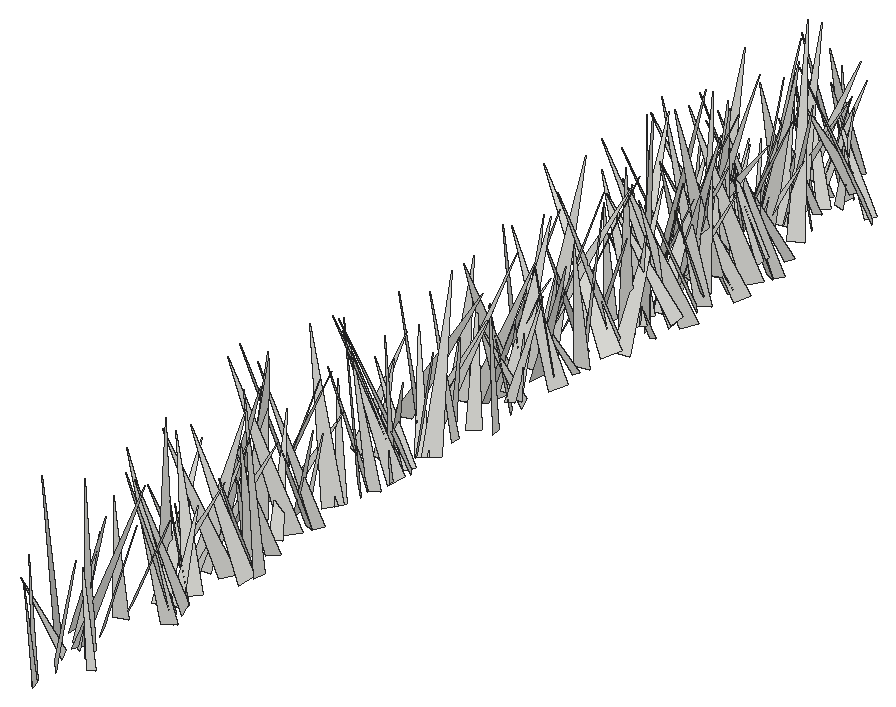
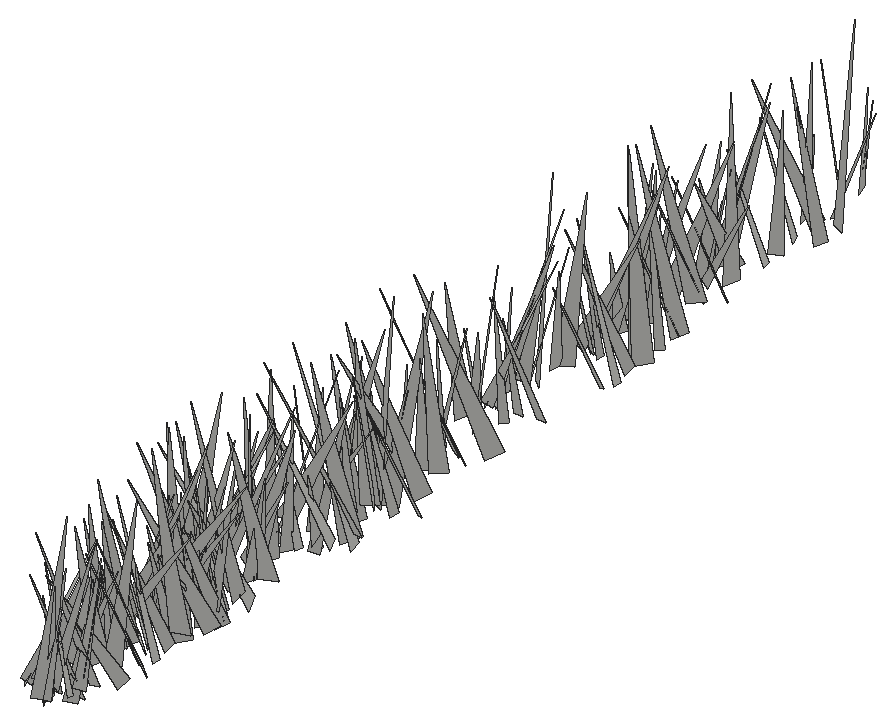
# SketchUp Ruby script. Lengths in inches.
U = 1.inch
M = Sketchup.active_model
def pt(a) = Geom::Point3d.new(a.map { |v| v * U })
def face(e, loops, mat)
  f = e.add_face(loops[0].map { |a| pt(a) })
  loops[1..].each { |l| e.add_face(l.map { |a| pt(a) }).erase! }
  f.material = f.back_material = mat if mat
  f
end
# faces: each face lists its corners as indices into pts; further lists are holes
def faces(e, pts, list, mat = nil) = list.each { |f| face(e, (f[0].is_a?(Array) ? f : [f]).map { |l| l.map { |i| pts[i] } }, mat) }
# xy, xz, yz: faces in a plane at the given z, y or x. An outline is a flat list of corners, or four numbers for a rectangle; further outlines are holes
def ring(l) = l.size == 4 ? [[l[0], l[1]], [l[2], l[1]], [l[2], l[3]], [l[0], l[3]]] : l.each_slice(2).to_a
def flat(e, list, mat, &to3) = list.each { |f| face(e, (f[0].is_a?(Array) ? f : [f]).map { |l| ring(l).map { |u, v| to3.(u, v) } }, mat) }
def xy(e, z, list, mat = nil) = flat(e, list, mat) { |x, y| [x, y, z] }
def xz(e, y, list, mat = nil) = flat(e, list, mat) { |x, z| [x, y, z] }
def yz(e, x, list, mat = nil) = flat(e, list, mat) { |y, z| [x, y, z] }
def lines(e, pts, list) = list.each { |a, b| e.add_line(pt(pts[a]), pt(pts[b])) }
# prism: a flat outline (further loops are holes) pulled along v
def prism(e, loops, v, mat = nil)
  f = face(e, loops, mat); d = Geom::Vector3d.new(v.map { |x| x * U })
  f.pushpull(f.normal.samedirection?(d) ? d.length : -d.length)
end
def box(e, o, s, mat = nil) = prism(e, [[o, [o[0] + s[0], o[1], o[2]], [o[0] + s[0], o[1] + s[1], o[2]], [o[0], o[1] + s[1], o[2]]]], [0, 0, s[2]], mat)
def at(x, y, z, deg = 0) = Geom::Transformation.translation(pt([x, y, z])) * Geom::Transformation.rotation(ORIGIN, Z_AXIS, deg.degrees)
def axes(o, x, y, z) = Geom::Transformation.new([*x, 0, *y, 0, *z, 0, *pt(o).to_a, 1])
def part(name) = M.definitions.add(name)
# library, detail: a bought-in or finely detailed component or shape, given as its bounding box
def library(name, o, s) = part(name).tap { |d| box(d.entities, o, s) }
def detail(e, o, s) = box(e.add_group.entities, o, s)
def put(e, d, t, mat = nil) = e.add_instance(d, t).tap { |i| i.material = mat if mat }
def group(e, t, mat = nil) = e.add_group.tap { |g| g.transformation = t; g.material = mat if mat }.entities
root = M.entities
c1 = part("fur_instance\#9")
p = [[0.8125,0,1.79],[0.67,-0.02,1.48],[0,-0.11,0],[0,0.11,0]]
faces(c1.entities,p,[[0,1,2,3]])
put(root,c1,axes([156.08,12.375,-27.1],[-3.70453,-1.18645,1.17686],[-1.32576,3.8289,-0.31316],[1.01735,0.66938,3.87726]))
put(root,c1,axes([155.93,12.61,-27.1],[-4.75488,-0.89522,1.48594],[-1.16705,4.85843,-0.80746],[1.28353,1.10117,4.77057]))
put(root,c1,axes([155.54,15.5,-27.1],[4.29125,3.34973,1.68987],[3.74545,-3.97458,-1.63261],[-0.21889,-2.33948,5.19327]))
put(root,c1,axes([154.88,17.29,-27.1],[-4.05266,-1.43323,0.72397],[-1.06557,3.87082,1.69814],[1.20119,-1.40176,3.94899]))
put(root,c1,axes([153.71,18.23,-27.1],[-3.953,-6.85404,2.35159],[-6.87911,4.39144,1.23577],[2.27722,1.36799,7.81517]))
put(root,c1,axes([157.96,16.73,-27.1],[-0.43735,3.78387,0.74816],[3.7266,0.2203,1.06426],[-0.99494,-0.83814,3.65736]))
put(root,c1,axes([156.37,18.52,-27.1],[-6.67663,-0.80436,2.4344],[-1.05353,7.05179,-0.55944],[2.33738,0.88086,6.7016]))
put(root,c1,axes([154.84,18.81,-27.1],[2.00613,4.44684,1.43472],[4.67253,-1.91449,-0.59961],[-0.01581,-1.5549,4.84142]))
put(root,c1,axes([153.21,20.83,-27.1],[6.29896,-1.22347,0.37639],[-1.1888,-6.29213,-0.55798],[-0.47466,-0.47719,6.39237]))
put(root,c1,axes([155.03,18.8,-27.1],[6.92746,0.46404,1.30725],[0.06508,-6.75935,2.05449],[-1.38564,2.00246,6.63205]))
put(root,c1,axes([155.05,21.61,-27.1],[4.65489,2.00226,0.76997],[2.06003,-4.68544,-0.26978],[-0.59848,-0.55448,5.06006]))
put(root,c1,axes([154.79,24.13,-27.1],[1.69924,-5.28596,1.58911],[-5.50046,-1.7602,0.02657],[-0.46001,1.5213,5.5523]))
put(root,c1,axes([157.84,26.63,-27.1],[-5.81163,-3.8947,1.27527],[-3.71182,5.94036,1.22659],[1.73708,-0.33677,6.88761]))
put(root,c1,axes([158.12,25.65,-27.1],[-0.65544,-6.57541,2.82853],[-6.91722,-0.14862,-1.94837],[-1.84083,2.89967,6.31422]))
put(root,c1,axes([154.35,25.83,-27.1],[4.46845,1.48023,0.19389],[1.49287,-4.43008,-0.58427],[0.00126,-0.6156,4.67084]))
put(root,c1,axes([157.67,28.15,-27.1],[-5.8236,-1.97497,1.08531],[-1.72724,5.8434,1.36532],[1.44743,-0.9731,5.99589]))
put(root,c1,axes([156.89,28.11,-27.1],[-2.21972,3.26489,1.22418],[3.2229,2.47495,-0.75684],[1.3308,-0.54808,3.87477]))
put(root,c1,axes([154.65,29.53,-27.1],[7.21029,-1.27081,2.71678],[-1.16788,-7.70491,-0.50453],[-2.76259,-0.05954,7.30402]))
put(root,c1,axes([157.25,28.9,-27.1],[2.56501,3.25674,2.5986],[3.3721,-3.41499,0.95138],[-2.44704,-1.29222,4.03491]))
put(root,c1,axes([156.14,30.48,-27.1],[-2.17091,-2.72609,1.07786],[-2.90812,2.17161,-0.36485],[0.36901,1.07644,3.46573]))
put(root,c1,axes([156.77,30.1,-27.1],[-4.49758,4.50366,1.60112],[4.72062,4.53017,0.51777],[0.74986,-1.50644,6.34374]))
put(root,c1,axes([156.125,30.83,-27.1],[-1.77005,-3.87903,0.89181],[-3.77258,1.32393,-1.7292],[-1.26879,1.475,3.89741]))
put(root,c1,axes([155.77,27.53,-27.1],[-5.23053,3.77379,0.03544],[3.44734,4.80229,-2.57973],[1.53577,2.07308,5.91142]))
put(root,c1,axes([153.26,31.82,-27.1],[3.75203,3.55416,0.24846],[3.4305,-3.50645,-1.64561],[0.96201,-1.35805,4.89916]))
put(root,c1,axes([157.1,33.93,-27.1],[2.35436,-6.19743,2.05043],[-5.78585,-2.99044,-2.39512],[-3.02263,0.89697,6.18179]))
put(root,c1,axes([158.5,34.32,-27.1],[-6.51837,1.52305,1.37348],[1.82295,6.39951,1.5551],[0.93967,-1.84981,6.5108]))
put(root,c1,axes([154.86,33.41,-27.1],[3.44666,-5.98968,2.82803],[-6.61551,-2.95389,1.80641],[0.33028,3.33943,6.67028]))
put(root,c1,axes([154.86,32.79,-27.1],[3.10305,4.72146,0.30771],[4.72969,-3.10544,-0.04628],[-0.13026,-0.28259,5.64969]))
put(root,c1,axes([156.52,36.87,-27.1],[-1.70648,-4.83175,0.15849],[-4.67215,1.69151,1.26205],[1.24174,-0.27565,4.96639]))
put(root,c1,axes([156.48,37.31,-27.1],[5.03393,-2.19184,1.50174],[-1.99616,-5.24318,-0.96135],[-1.75349,-0.32355,5.40559]))
put(root,c1,axes([155.66,37.99,-27.1],[4.05773,-0.76512,0.97615],[-0.40955,-3.97873,-1.41614],[-1.1707,-1.26007,3.87881]))
put(root,c1,axes([158.76,35.45,-27.1],[-7.01031,-0.43579,1.43561],[-0.72042,6.99511,-1.39453],[1.31601,1.50792,6.88401]))
put(root,c1,axes([157.57,38.55,-27.1],[1.87791,-4.76016,0.94457],[-4.63856,-2.05833,-1.15104],[-1.42657,0.4266,4.98606]))
put(root,c1,axes([152.66,38.09,-27.1],[7.35605,-1.97253,1.00478],[-2.03855,-7.39535,0.40615],[-0.86301,0.65556,7.60509]))
put(root,c1,axes([152.83,38.13,-27.1],[3.6305,3.98779,0.322],[3.84064,-3.3521,-1.78874],[1.12055,-1.43096,5.08758]))
put(root,c1,axes([152.55,40.58,-27.1],[6.00758,0.21792,0.49644],[0.387,-5.59183,-2.22857],[-0.3797,-2.2514,5.58318]))
put(root,c1,axes([156.76,41.83,-27.1],[2.25381,-7.00366,2.80187],[-6.80723,-3.14832,-2.39397],[-3.25014,1.7373,6.957]))
put(root,c1,axes([153.15,42.1,-27.1],[4.39252,-6.51911,2.0007],[-6.79057,-4.39945,0.57342],[-0.62428,1.98542,7.83991]))
put(root,c1,axes([152.14,43.08,-27.1],[7.73764,-3.02475,0.93063],[-2.93122,-7.77665,-0.90436],[-1.19293,-0.51074,8.25847]))
put(root,c1,axes([156.38,40.4,-27.1],[-4.08982,2.78235,0.32679],[2.66533,4.04258,-1.06229],[0.86271,0.7007,4.83111]))
put(root,c1,axes([157.04,43.43,-27.1],[-4.74845,-6.02691,1.04144],[-6.05438,4.44477,-1.88271],[-0.8676,1.96887,7.4382]))
put(root,c1,axes([155.16,44.26,-27.1],[4.1341,0.32333,0.78637],[0.3951,-4.18703,-0.35553],[-0.75288,-0.42186,4.13146]))
put(root,c1,axes([157.69,43.76,-27.1],[-2.26256,-5.81888,2.33683],[-5.71547,0.89178,-3.31322],[-2.57945,3.12805,5.2916]))
put(root,c1,axes([156.18,43.99,-27.1],[1.71748,3.11444,0.84575],[3.20742,-1.75327,-0.057],[-0.35706,-0.7688,3.55615]))
put(root,c1,axes([152.29,44.39,-27.1],[6.26365,0.83218,0.34032],[0.77044,-6.2027,0.98722],[-0.46342,0.93576,6.24109]))
put(root,c1,axes([151.74,46.61,-27.1],[6.21728,1.67139,0.47713],[1.73743,-6.02723,-1.52629],[-0.05031,-1.59834,6.25448]))
put(root,c1,axes([156.51,46.92,-27.1],[-5.45216,4.70878,2.71596],[5.23215,5.58914,0.81316],[1.47433,-2.42158,7.15803]))
put(root,c1,axes([152.3,47.71,-27.1],[2.38056,3.51502,0.37387],[3.33138,-2.08023,-1.65431],[1.18197,-1.21634,3.90969]))
put(root,c1,axes([156.83,47.42,-27.1],[-4.5869,1.43943,1.05541],[1.33614,4.69877,-0.60151],[1.18347,0.27406,4.76967]))
put(root,c1,axes([156.39,50.14,-27.1],[-5.2101,-5.93708,2.74108],[-5.84341,5.80017,1.45611],[2.93548,1.00834,7.76362]))
put(root,c1,axes([156.6,50.95,-27.1],[-4.48519,-3.52054,0.94744],[-3.42145,4.58335,0.83384],[1.25916,-0.08621,5.64055]))
put(root,c1,axes([157.41,50.62,-27.1],[0.3865,-5.10308,2.42648],[-5.49086,-0.91339,-1.04632],[-1.33405,2.28099,5.00959]))
put(root,c1,axes([157.76,52.81,-27.1],[-5.95975,2.47486,1.75961],[2.91321,5.75356,1.77469],[0.85695,-2.34763,6.20435]))
put(root,c1,axes([156.88,54.54,-27.1],[-5.73536,-5.62008,0.65862],[-5.46135,5.74328,1.44982],[1.48081,-0.58562,7.89796]))
put(root,c1,axes([157.61,54.76,-27.1],[-5.40162,-4.18627,0.13743],[-4.18531,5.38577,-0.4449],[-0.16419,0.43574,6.81941]))
put(root,c1,axes([157.625,52.58,-27.1],[-5.30333,-1.20318,1.41609],[-1.56427,5.2022,-1.4382],[1.00301,1.75149,5.24448]))
put(root,c1,axes([154.6,56.35,-27.1],[4.66467,-0.77947,0.02704],[-0.7406,-4.47818,-1.32848],[-0.24456,-1.30606,4.53893]))
put(root,c1,axes([154.5625,54.71,-27.1],[0.69151,3.97199,1.28395],[4.17346,-0.6309,-0.296],[0.08642,-1.31479,4.02085]))
put(root,c1,axes([157.38,54.89,-27.1],[-1.85647,3.95367,0.8299],[3.82368,1.42492,1.76516],[-1.30372,-1.4508,3.99527]))
put(root,c1,axes([152.72,54.29,-27.1],[2.02103,5.13059,0.73898],[5.12624,-1.86067,-1.10143],[0.76856,-1.08099,5.40318]))
put(root,c1,axes([155.69,58.44,-27.1],[-5.52938,-3.456,2.07939],[-3.45701,5.87854,0.57763],[2.07771,0.58365,6.49494]))
put(root,c1,axes([156.48,56.83,-27.1],[3.3556,2.16226,1.21696],[2.08771,-3.56664,0.58052],[-1.34083,-0.14202,3.94948]))
put(root,c1,axes([156.95,56.85,-27.1],[-1.86757,4.60063,0.33127],[4.58089,1.80817,0.71369],[-0.53944,-0.57279,4.91369]))
put(root,c1,axes([157.47,57.34,-27.1],[-5.92088,3.75972,1.43779],[3.50525,6.07307,-1.44586],[1.97886,0.49178,6.86307]))
put(root,c1,axes([152.07,60.59,-27.1],[6.07863,-4.42165,0.21276],[-4.21796,-5.67554,2.55792],[1.3435,2.18706,7.06807]))
put(root,c1,axes([157.35,60.24,-27.1],[-5.62081,-1.07857,0.79033],[-1.22962,5.511,-1.22409],[0.52534,1.35906,5.59093]))
put(root,c1,axes([156,61.7,-27.1],[-1.72893,-3.46771,1.76985],[-3.62718,2.13831,0.64633],[1.41454,1.24466,3.82053]))
put(root,c1,axes([153.01,62.92,-27.1],[3.55975,3.91646,0.08522],[3.79537,-3.41954,-1.38552],[0.97011,-0.99289,5.10792]))
put(root,c1,axes([154.51,62.12,-27.1],[4.64022,6.0526,0.40907],[6.0581,-4.59639,-0.71102],[0.31728,-0.75645,7.59342]))
put(root,c1,axes([156.15,63.97,-28.22],[-3.13208,3.88614,1.48189],[4.03166,3.29255,-0.11327],[1.02167,-1.07935,4.98991]))
put(root,c1,axes([153.67,65.17,-27.1],[3.4619,-5.09824,2.22403],[-5.52391,-3.4582,0.67108],[-0.65172,2.22978,6.12588]))
put(root,c1,axes([157.64,64.65,-28.22],[-4.75488,-0.89522,1.48594],[-1.16705,4.85843,-0.80746],[1.28353,1.10117,4.77057]))
put(root,c1,axes([154.83,69.78,-28.22],[6.488,-4.94571,0.82766],[-4.48999,-6.33233,-2.64212],[-2.23271,-1.63731,7.71838]))
put(root,c1,axes([156.59,69.34,-28.22],[-4.05266,-1.43323,0.72397],[-1.06557,3.87082,1.69814],[1.20119,-1.40176,3.94899]))
put(root,c1,axes([156.57,67.83,-28.22],[-3.48684,-2.54111,1.02639],[-2.66037,3.53733,-0.28017],[0.65812,0.83597,4.30544]))
put(root,c1,axes([153.56,67.2,-28.22],[6.12264,-2.56902,1.18593],[-2.80714,-5.86992,1.77677],[-0.35534,2.10644,6.39763]))
put(root,c1,axes([155.43,70.27,-28.22],[-3.953,-6.85404,2.35159],[-6.87911,4.39144,1.23577],[2.27722,1.36799,7.81517]))
put(root,c1,axes([156.87,67.3,-27.1],[3.7026,-0.58317,1.91769],[-1.4169,-3.61072,1.63767],[-1.41775,2.08554,3.37155]))
put(root,c1,axes([157.23,67.87,-27.1],[1.77865,4.09096,1.0407],[3.89915,-2.02489,1.29578],[-1.61729,-0.38272,4.26855]))
put(root,c1,axes([156.2,68.3,-27.1],[-1.91497,6.86191,1.78883],[6.91485,2.21764,-1.10438],[1.57179,-1.39609,7.03799]))
put(root,c1,axes([151.95,69.55,-28.22],[4.10846,4.74791,0.21399],[4.46685,-3.7608,-2.31765],[1.62348,-1.66782,5.83529]))
put(root,c1,axes([153.53,70.57,-28.22],[5.27208,0.02621,0.0042],[0.02652,-5.23568,-0.61848],[-0.0011,-0.61849,5.23574]))
put(root,c1,axes([155.48,66.15,-27.1],[6.83312,3.40706,1.30672],[2.45514,-6.34476,3.70451],[-2.69961,2.8536,6.67654]))
put(root,c1,axes([158.37,71.16,-27.1],[-6.07802,2.92755,1.98205],[3.37511,5.97833,1.51972],[1.05246,-2.26504,6.57292]))
put(root,c1,axes([156.44,72.91,-27.1],[-3.5454,-4.09399,1.47684],[-3.82101,3.83994,1.47185],[2.08366,0.07566,5.21193]))
put(root,c1,axes([154.62,72.05,-27.1],[3.53738,-5.32848,1.99163],[-5.66565,-3.51029,0.67133],[-0.50966,2.039,6.36044]))
put(root,c1,axes([154.92,72.87,-28.22],[6.29896,-1.22347,0.37639],[-1.1888,-6.29213,-0.55798],[-0.47466,-0.47719,6.39237]))
put(root,c1,axes([158,73.67,-27.1],[-0.53868,-3.7535,0.51973],[-3.36849,0.23389,-1.80211],[-1.73555,0.71104,3.33637]))
put(root,c1,axes([154.36,71.85,-27.1],[4.62309,3.63215,1.82021],[3.50208,-4.96051,1.00367],[-2.05939,-0.28182,5.79293]))
put(root,c1,axes([154.83,74.04,-27.1],[4.24921,-1.39082,0.67887],[-1.35455,-4.30166,-0.33452],[-0.74864,-0.11098,4.4585]))
put(root,c1,axes([156.5,76.17,-28.22],[1.69924,-5.28596,1.58911],[-5.50046,-1.7602,0.02657],[-0.46001,1.5213,5.5523]))
put(root,c1,axes([154.6,78.69,-28.22],[-1.67702,-6.45132,0.05531],[-6.32349,1.655,1.30744],[1.27907,-0.27646,6.53625]))
put(root,c1,axes([152.79,76.13,-28.22],[7.89024,2.57718,0.73013],[2.64489,-7.85516,-0.85554],[-0.42369,-1.04189,8.25626]))
put(root,c1,axes([153.55,75.58,-28.22],[6.54564,-3.57049,3.76512],[-4.66006,-6.71077,1.73761],[-2.28219,3.46223,7.25083]))
put(root,c1,axes([156.35,76.74,-27.1],[3.88828,4.27161,1.82836],[4.44707,-4.1121,0.14976],[-1.3465,-1.2459,5.77433]))
put(root,c1,axes([157.6,79.02,-27.1],[-6.20771,-3.16783,0.82777],[-3.08728,6.25411,0.78157],[1.09042,-0.32718,6.92531]))
put(root,c1,axes([152.47,76.18,-27.1],[3.82071,6.83533,0.31448],[6.59967,-3.58608,-2.23672],[1.80694,-1.35528,7.50444]))
put(root,c1,axes([158.22,77.51,-27.1],[-5.28258,5.45364,0.12335],[5.18528,4.96674,2.47132],[-1.69419,-1.80343,7.17917]))
put(root,c1,axes([154.81,78.01,-28.22],[-2.61192,2.51011,0.78878],[2.46687,2.72278,-0.49597],[0.91509,-0.17543,3.58843]))
put(root,c1,axes([154.54,80.54,-27.1],[5.4983,0.81734,0.21266],[0.84397,-5.26527,-1.58403],[0.03145,-1.59793,5.32824]))
put(root,c1,axes([153.01,78.48,-27.1],[6.48449,2.8801,0.19854],[2.8437,-6.45643,0.78158],[-0.49773,0.63448,7.05214]))
put(root,c1,axes([155.1,81.3,-27.1],[-4.81176,0.83188,2.6308],[1.27412,5.3609,0.63523],[2.44739,-1.15538,4.84165]))
put(root,c1,axes([156.36,81.57,-28.22],[7.21029,-1.27081,2.71678],[-1.16788,-7.70491,-0.50453],[-2.76259,-0.05954,7.30402]))
put(root,c1,axes([157.14,82.03,-27.1],[-2.40654,5.51072,1.54274],[5.60544,1.9331,1.83892],[-1.15197,-2.10585,5.72519]))
put(root,c1,axes([157.84,82.875,-28.22],[-1.77005,-3.87903,0.89181],[-3.77258,1.32393,-1.7292],[-1.26879,1.475,3.89741]))
put(root,c1,axes([157.48,79.57,-28.22],[-5.23053,3.77379,0.03544],[3.44734,4.80229,-2.57973],[1.53577,2.07308,5.91142]))
put(root,c1,axes([155.92,83.32,-27.1],[0.94774,-3.5048,1.15841],[-3.67796,-0.79512,0.60341],[0.31324,1.26803,3.58018]))
put(root,c1,axes([158.84,84.41,-27.1],[-5.67147,0.82087,0.04901],[0.80443,5.46726,1.5178],[-0.17066,-1.50898,5.5259]))
put(root,c1,axes([157.63,85.64,-27.1],[-4.78026,1.17069,2.19317],[1.89155,4.79719,1.56216],[1.61324,-2.15588,4.66702]))
put(root,c1,axes([158.8125,85.97,-28.22],[2.35436,-6.19743,2.05043],[-5.78585,-2.99044,-2.39512],[-3.02263,0.89697,6.18179]))
put(root,c1,axes([157.71,85.77,-28.22],[-8.03194,-0.35365,0.82088],[-0.22203,7.97883,1.26494],[0.86581,-1.23463,7.93959]))
put(root,c1,axes([157.08,82.81,-27.1],[-7.37531,-1.40171,2.74866],[-2.16749,7.42249,-2.03071],[2.19589,2.61858,7.22747]))
put(root,c1,axes([155.46,84.07,-28.22],[-4.82421,0.67017,1.12309],[0.52178,4.9221,-0.69578],[1.19925,0.5543,4.82058]))
put(root,c1,axes([156.76,83.58,-28.22],[-7.31055,-2.64435,2.80127],[-3.45475,7.15889,-2.25809],[1.70424,3.16886,7.43894]))
put(root,c1,axes([155.64,85.04,-28.22],[-4.87029,1.64927,0.93909],[1.65484,4.95663,-0.12272],[0.92923,-0.18296,5.1405]))
put(root,c1,axes([158.81,86.8,-27.1],[-5.4011,-4.4458,0.12135],[-4.40164,5.31613,-1.14717],[-0.63674,0.96192,6.9008]))
put(root,c1,axes([154.6875,84.01,-28.22],[-2.31741,7.72302,0.72504],[7.71845,2.37113,-0.58682],[0.77216,-0.52327,8.04183]))
put(root,c1,axes([157.83,88.68,-27.1],[-2.17535,-3.01047,0.60266],[-3.06621,2.16789,-0.23847],[0.15643,0.62897,3.70651]))
put(root,c1,axes([154.89,86.74,-28.22],[3.77893,2.89431,1.05154],[2.64296,-3.90266,1.24382],[-1.58036,0.3941,4.59459]))
put(root,c1,axes([156.66,91.37,-27.1],[1.61042,-7.88282,1.5376],[-7.97737,-1.75156,-0.62458],[-0.92985,1.37466,8.02136]))
put(root,c1,axes([153.78,91.58,-27.1],[-0.77388,-5.77446,0.46112],[-5.72229,0.83441,0.84559],[0.90132,0.33953,5.76439]))
put(root,c1,axes([157.74,88.95,-28.22],[-0.49595,7.7495,2.67586],[7.77568,-0.40515,2.61451],[-2.59882,-2.6911,7.31198]))
put(root,c1,axes([155.89,86.18,-28.22],[-5.33853,3.8285,0.2094],[3.37353,4.86067,-2.86257],[1.82225,2.21756,5.91295]))
put(root,c1,axes([153.49,88.93,-27.1],[8.05424,1.38868,1.7961],[1.29513,-8.24767,0.56905],[-1.86468,0.26973,8.15325]))
put(root,c1,axes([154.37,90.13,-28.22],[7.35605,-1.97253,1.00478],[-2.03855,-7.39535,0.40615],[-0.86301,0.65556,7.60509]))
put(root,c1,axes([153.42,87.5,-28.22],[7.40987,3.38689,0.1989],[3.26816,-7.25381,1.76579],[-0.91088,1.52574,7.95356]))
put(root,c1,axes([153.31,90.64,-28.22],[5.88028,2.97965,0.94292],[3.11911,-5.72141,-1.37172],[-0.19635,-1.65292,6.44782]))
put(root,c1,axes([154.54,90.17,-28.22],[3.6305,3.98779,0.322],[3.84064,-3.3521,-1.78874],[1.12055,-1.43096,5.08758]))
put(root,c1,axes([154.26,92.62,-28.22],[6.00758,0.21792,0.49644],[0.387,-5.59183,-2.22857],[-0.3797,-2.2514,5.58318]))
put(root,c1,axes([157.57,89.2,-27.1],[1.24745,7.40868,1.63783],[7.39275,-1.56046,1.42803],[-1.70827,-1.34297,7.376]))
put(root,c1,axes([155.36,91.9,-27.1],[0.47741,-4.86513,1.33169],[-4.92648,-0.73691,-0.92606],[-1.08291,1.20759,4.79999]))
put(root,c1,axes([154.91,91.61,-28.22],[-2.5079,-4.6968,1.95628],[-4.90602,2.8103,0.45782],[1.34828,1.48955,5.3047]))
put(root,c1,axes([155.43,89.94,-27.1],[2.35955,4.93164,1.36493],[4.86886,-2.62618,1.07189],[-1.57426,-0.73054,5.36093]))
put(root,c1,axes([158.19,91.73,-28.22],[-2.71557,-5.16024,0.69315],[-4.67023,2.06855,-2.89705],[-2.30163,1.89099,5.06058]))
put(root,c1,axes([159.3,91.57,-28.22],[-2.51256,7.06983,2.10699],[6.38069,0.96553,4.36915],[-3.70253,-3.13371,6.09968]))
put(root,c1,axes([155.25,92.01,-27.1],[-0.48209,-3.49328,1.24378],[-3.69826,0.54426,0.09516],[0.26993,1.21786,3.5251]))
put(root,c1,axes([153,91.48,-28.22],[5.01849,-2.22986,0.6447],[-2.32023,-4.77497,1.54574],[0.06662,1.67347,5.26955]))
put(root,c1,axes([156.18,92.16,-27.1],[-2.69115,3.5868,1.84623],[3.86426,2.92918,-0.05799],[1.15809,-1.43902,4.48375]))
put(root,c1,axes([158.47,93.87,-28.22],[2.25381,-7.00366,2.80187],[-6.80723,-3.14832,-2.39397],[-3.25014,1.7373,6.957]))
put(root,c1,axes([154.86,94.14,-28.22],[4.39252,-6.51911,2.0007],[-6.79057,-4.39945,0.57342],[-0.62428,1.98542,7.83991]))
put(root,c1,axes([153.85,95.12,-28.22],[7.73764,-3.02475,0.93063],[-2.93122,-7.77665,-0.90436],[-1.19293,-0.51074,8.25847]))
put(root,c1,axes([155.43,90.64,-27.1],[7.73551,0.03019,2.73159],[-1.01366,-7.58581,2.95441],[-2.53672,3.12332,7.14916]))
put(root,c1,axes([153.98,91.16,-28.22],[3.66299,2.22216,0.32756],[1.7102,-3.16536,2.34915],[-1.4562,1.87225,3.58288]))
put(root,c1,axes([157.27,94.55,-27.1],[-3.81411,-2.18756,1.38745],[-2.30966,3.98998,-0.05835],[1.17299,0.74331,4.39652]))
put(root,c1,axes([151.97,93.98,-27.1],[4.55,-4.60588,0.41001],[-4.16176,-3.82822,3.1795],[2.01545,2.49305,5.6398]))
put(root,c1,axes([158.24,95.29,-27.1],[-5.1344,0.67452,1.09766],[0.89094,5.11676,1.02317],[0.93062,-1.17714,5.07643]))
put(root,c1,axes([158.75,95.47,-28.22],[-4.74845,-6.02691,1.04144],[-6.05438,4.44477,-1.88271],[-0.8676,1.96887,7.4382]))
put(root,c1,axes([156.93,93.9375,-28.22],[-1.00856,5.27208,0.80529],[5.17147,0.76643,1.45913],[-1.30357,-1.0384,5.16556]))
put(root,c1,axes([156.04,93.125,-28.22],[-4.2837,1.86088,0.37109],[1.60299,4.03921,-1.75094],[1.01537,1.47394,4.32979]))
put(root,c1,axes([155.22,94.09,-28.22],[-2.74828,4.07366,1.32335],[3.94461,3.01992,-1.10419],[1.66916,-0.42944,4.78838]))
put(root,c1,axes([159.4,95.8,-28.22],[-2.26256,-5.81888,2.33683],[-5.71547,0.89178,-3.31322],[-2.57945,3.12805,5.2916]))
put(root,c1,axes([153.48,95.85,-27.1],[-0.77106,7.66776,2.67234],[8.04873,1.0768,-0.76736],[1.07416,-2.56446,7.66813]))
put(root,c1,axes([154.64,95.57,-27.1],[-1.99149,3.68652,0.84504],[3.6319,2.13053,-0.73532],[1.05538,-0.37542,4.12502]))
put(root,c1,axes([158.42,98.3,-28.22],[-1.84266,-5.86998,0.99209],[-5.21002,1.08759,-3.24178],[-2.88039,1.78795,5.22904]))
put(root,c1,axes([154,96.43,-28.22],[6.26365,0.83218,0.34032],[0.77044,-6.2027,0.98722],[-0.46342,0.93576,6.24109]))
put(root,c1,axes([153.45,98.65,-28.22],[6.21728,1.67139,0.47713],[1.73743,-6.02723,-1.52629],[-0.05031,-1.59834,6.25448]))
put(root,c1,axes([156.83,96.125,-27.1],[0.48963,4.22721,0.04806],[3.94805,-0.47454,1.51627],[-1.51146,0.12987,3.97618]))
put(root,c1,axes([155.8,96.88,-28.22],[4.5947,4.98178,1.41698],[4.55399,-4.78808,2.06705],[-2.46722,0.43974,6.4542]))
put(root,c1,axes([154.01,99.75,-28.22],[2.38056,3.51502,0.37387],[3.33138,-2.08023,-1.65431],[1.18197,-1.21634,3.90969]))
put(root,c1,axes([155.25,99.4,-27.1],[6.61649,-1.70465,2.3436],[-2.13195,-6.81989,1.0584],[-1.96294,1.66119,6.75008]))
put(root,c1,axes([154.3,102.8,-27.1],[4.71186,-4.25626,1.34995],[-4.06485,-4.9009,-1.26409],[-1.848,-0.07223,6.22249]))
put(root,c1,axes([155.93,101.04,-27.1],[5.31059,0.52385,1.16283],[0.52648,-5.43598,0.04446],[-1.16164,-0.06886,5.33618]))
put(root,c1,axes([155.65,100.35,-27.1],[-2.00411,5.21831,1.67163],[5.38658,2.20263,-0.41796],[1.00489,-1.39973,5.57427]))
put(root,c1,axes([154.46,102.63,-27.1],[0.84418,-3.62493,0.18375],[-3.45271,-0.74384,1.18829],[1.11924,0.43944,3.52714]))
put(root,c1,axes([155.8,97.3125,-28.22],[4.35175,7.0169,0.44581],[6.16578,-4.0605,3.72408],[-3.37917,1.6275,7.36925]))
put(root,c1,axes([158.23,99.24,-27.1],[0.30584,8.28043,0.48557],[7.987,-0.4251,2.21855],[-2.2381,-0.38549,7.98355]))
put(root,c1,axes([153.13,100.45,-28.22],[3.77289,4.9439,0.17652],[4.9129,-3.7705,0.5956],[-0.58026,0.22179,6.19049]))
put(root,c1,axes([156.9,103.43,-27.1],[-0.5806,-4.0301,0.94816],[-3.96701,0.26756,-1.29192],[-1.18471,1.07913,3.86131]))
put(root,c1,axes([156.68,102.97,-28.22],[-3.71707,-2.68533,1.32909],[-2.9797,3.53518,-1.19076],[0.31439,1.75658,4.42828]))
put(root,c1,axes([153.25,102.76,-28.22],[5.52796,-0.81869,0.7417],[-1.07099,-4.89962,2.57397],[-0.27083,2.66498,4.96017]))
put(root,c1,axes([155.375,102.9,-27.1],[-6.19625,3.45387,1.64148],[3.0912,6.3638,-1.72156],[2.25127,0.76815,6.88178]))
put(root,c1,axes([155.24,104.88,-27.1],[-4.18009,-2.38384,1.39005],[-2.61185,4.23208,-0.59649],[0.8906,1.22265,4.77494]))
put(root,c1,axes([154.01,107.03,-27.1],[0.47232,-5.02453,0.37853],[-5.03579,-0.45765,0.20889],[0.17316,0.39615,5.04235]))
put(root,c1,axes([156.79,104.26,-27.1],[-1.63602,4.97918,0.62205],[4.87533,1.42244,1.43652],[-1.18757,-1.0199,5.04036]))
put(root,c1,axes([157.19,107.78,-27.1],[2.87484,-4.36178,0.57915],[-3.91954,-2.85297,-2.03053],[-1.99945,-0.67874,4.81319]))
put(root,c1,axes([159.32,106.8,-28.22],[-5.40162,-4.18627,0.13743],[-4.18531,5.38577,-0.4449],[-0.16419,0.43574,6.81941]))
put(root,c1,axes([154.59,107.35,-28.22],[2.25117,-4.50739,0.41367],[-4.42833,-2.28883,-0.84056],[-0.93676,-0.01195,4.96767]))
put(root,c1,axes([153.51,105.82,-27.1],[2.52048,5.79703,1.2985],[5.75928,-2.03853,-2.07834],[1.45681,-1.97061,5.96983]))
put(root,c1,axes([156.27,106.75,-28.22],[0.69151,3.97199,1.28395],[4.17346,-0.6309,-0.296],[0.08642,-1.31479,4.02085]))
put(root,c1,axes([155.9,107.72,-27.1],[-2.90009,-5.61636,1.60668],[-5.82709,2.65472,-1.23809],[-0.41218,1.98605,6.19848]))
put(root,c1,axes([159.09,106.93,-28.22],[-1.85647,3.95367,0.8299],[3.82368,1.42492,1.76516],[-1.30372,-1.4508,3.99527]))
put(root,c1,axes([153.88,108.26,-27.1],[4.89387,1.35478,0.49174],[1.44124,-4.60961,-1.64362],[-0.00784,-1.71558,4.80457]))
put(root,c1,axes([154.43,106.34,-28.22],[2.02103,5.13059,0.73898],[5.12624,-1.86067,-1.10143],[0.76856,-1.08099,5.40318]))
put(root,c1,axes([155.28,109.91,-27.1],[3.26606,-6.16963,0.62937],[-6.14796,-3.31446,-0.58694],[-0.81426,0.27855,6.95607]))
put(root,c1,axes([155.07,109.83,-27.1],[1.17594,-4.92519,0.34785],[-4.93492,-1.18388,-0.07952],[-0.1583,0.31979,5.06301]))
put(root,c1,axes([156.15,108.625,-28.22],[-2.57629,-2.49445,0.93197],[-2.62206,2.60252,-0.28257],[0.46438,0.85602,3.57488]))
put(root,c1,axes([156.06,108.03,-28.22],[-5.10853,0.04095,1.59169],[-0.11644,5.32521,-0.51071],[1.58796,0.52222,5.08311]))
